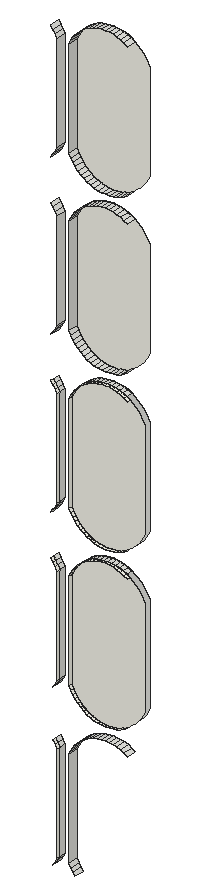
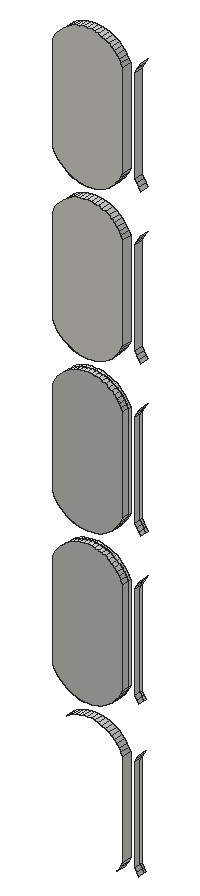
# SketchUp Ruby script. Lengths in inches.
U = 1.inch
M = Sketchup.active_model
def pt(a) = Geom::Point3d.new(a.map { |v| v * U })
def face(e, loops, mat)
  f = e.add_face(loops[0].map { |a| pt(a) })
  loops[1..].each { |l| e.add_face(l.map { |a| pt(a) }).erase! }
  f.material = f.back_material = mat if mat
  f
end
# faces: each face lists its corners as indices into pts; further lists are holes
def faces(e, pts, list, mat = nil) = list.each { |f| face(e, (f[0].is_a?(Array) ? f : [f]).map { |l| l.map { |i| pts[i] } }, mat) }
# xy, xz, yz: faces in a plane at the given z, y or x. An outline is a flat list of corners, or four numbers for a rectangle; further outlines are holes
def ring(l) = l.size == 4 ? [[l[0], l[1]], [l[2], l[1]], [l[2], l[3]], [l[0], l[3]]] : l.each_slice(2).to_a
def flat(e, list, mat, &to3) = list.each { |f| face(e, (f[0].is_a?(Array) ? f : [f]).map { |l| ring(l).map { |u, v| to3.(u, v) } }, mat) }
def xy(e, z, list, mat = nil) = flat(e, list, mat) { |x, y| [x, y, z] }
def xz(e, y, list, mat = nil) = flat(e, list, mat) { |x, z| [x, y, z] }
def yz(e, x, list, mat = nil) = flat(e, list, mat) { |y, z| [x, y, z] }
def lines(e, pts, list) = list.each { |a, b| e.add_line(pt(pts[a]), pt(pts[b])) }
# prism: a flat outline (further loops are holes) pulled along v
def prism(e, loops, v, mat = nil)
  f = face(e, loops, mat); d = Geom::Vector3d.new(v.map { |x| x * U })
  f.pushpull(f.normal.samedirection?(d) ? d.length : -d.length)
end
def box(e, o, s, mat = nil) = prism(e, [[o, [o[0] + s[0], o[1], o[2]], [o[0] + s[0], o[1] + s[1], o[2]], [o[0], o[1] + s[1], o[2]]]], [0, 0, s[2]], mat)
def at(x, y, z, deg = 0) = Geom::Transformation.translation(pt([x, y, z])) * Geom::Transformation.rotation(ORIGIN, Z_AXIS, deg.degrees)
def axes(o, x, y, z) = Geom::Transformation.new([*x, 0, *y, 0, *z, 0, *pt(o).to_a, 1])
def part(name) = M.definitions.add(name)
# library, detail: a bought-in or finely detailed component or shape, given as its bounding box
def library(name, o, s) = part(name).tap { |d| box(d.entities, o, s) }
def detail(e, o, s) = box(e.add_group.entities, o, s)
def put(e, d, t, mat = nil) = e.add_instance(d, t).tap { |i| i.material = mat if mat }
def group(e, t, mat = nil) = e.add_group.tap { |g| g.transformation = t; g.material = mat if mat }.entities
root = M.entities
M.materials.add("Tafisa-Gardenia-or-Gardenia-PM775-4K").color = [246, 245, 235]
xz(root,138.25,[[96.53,63,96.85,63.02,97.16,63.0625,97.47,63.14,97.76,63.25,98.05,63.38,98.32,63.55,98.57,63.74,98.81,63.95,99.02,64.19,99.21,64.44,99.37,64.71,99.5,65,99.5,73,99.37,73.29,99.21,73.56,99.02,73.81,98.81,74.05,98.57,74.26,98.32,74.45,98.05,74.62,97.76,74.75,97.47,74.86,97.16,74.9375,96.85,74.98,96.53,75,96.22,74.98,95.9,74.9375,95.6,74.86,95.3,74.75,95.01,74.62,94.74,74.45,94.49,74.26,94.25,74.05,94.04,73.81,93.86,73.56,93.7,73.29,93.5625,73,93.5625,65,93.7,64.71,93.86,64.44,94.04,64.19,94.25,63.95,94.49,63.74,94.74,63.55,95.01,63.38,95.3,63.25,95.6,63.14,95.9,63.0625,96.22,63.02],[96.53,76,96.85,76.02,97.16,76.0625,97.47,76.14,97.76,76.25,98.05,76.38,98.32,76.55,98.57,76.74,98.81,76.95,99.02,77.19,99.21,77.44,99.37,77.71,99.5,78,99.5,86,99.37,86.29,99.21,86.56,99.02,86.81,98.81,87.05,98.57,87.26,98.32,87.45,98.05,87.62,97.76,87.75,97.47,87.86,97.16,87.9375,96.85,87.98,96.53,88,96.22,87.98,95.9,87.9375,95.6,87.86,95.3,87.75,95.01,87.62,94.74,87.45,94.49,87.26,94.25,87.05,94.04,86.81,93.86,86.56,93.7,86.29,93.5625,86,93.5625,78,93.7,77.71,93.86,77.44,94.04,77.19,94.25,76.95,94.49,76.74,94.74,76.55,95.01,76.38,95.3,76.25,95.6,76.14,95.9,76.0625,96.22,76.02]],"Tafisa-Gardenia-or-Gardenia-PM775-4K")
xz(root,138.79,[[96.53,63,96.85,63.02,97.16,63.0625,97.47,63.14,97.76,63.25,98.05,63.38,98.32,63.55,98.57,63.74,98.81,63.95,99.02,64.19,99.21,64.44,99.37,64.71,99.5,65,99.5,73,99.37,73.29,99.21,73.56,99.02,73.81,98.81,74.05,98.57,74.26,98.32,74.45,98.05,74.62,97.76,74.75,97.47,74.86,97.16,74.9375,96.85,74.98,96.53,75,96.22,74.98,95.9,74.9375,95.6,74.86,95.3,74.75,95.01,74.62,94.74,74.45,94.49,74.26,94.25,74.05,94.04,73.81,93.86,73.56,93.7,73.29,93.5625,73,93.5625,65,93.7,64.71,93.86,64.44,94.04,64.19,94.25,63.95,94.49,63.74,94.74,63.55,95.01,63.38,95.3,63.25,95.6,63.14,95.9,63.0625,96.22,63.02],[96.53,76,96.85,76.02,97.16,76.0625,97.47,76.14,97.76,76.25,98.05,76.38,98.32,76.55,98.57,76.74,98.81,76.95,99.02,77.19,99.21,77.44,99.37,77.71,99.5,78,99.5,86,99.37,86.29,99.21,86.56,99.02,86.81,98.81,87.05,98.57,87.26,98.32,87.45,98.05,87.62,97.76,87.75,97.47,87.86,97.16,87.9375,96.85,87.98,96.53,88,96.22,87.98,95.9,87.9375,95.6,87.86,95.3,87.75,95.01,87.62,94.74,87.45,94.49,87.26,94.25,87.05,94.04,86.81,93.86,86.56,93.7,86.29,93.5625,86,93.5625,78,93.7,77.71,93.86,77.44,94.04,77.19,94.25,76.95,94.49,76.74,94.74,76.55,95.01,76.38,95.3,76.25,95.6,76.14,95.9,76.0625,96.22,76.02]])
xz(root,138.79,[[96.53,89,96.85,89.02,97.16,89.0625,97.47,89.14,97.76,89.25,98.05,89.38,98.32,89.55,98.57,89.74,98.81,89.95,99.02,90.19,99.21,90.44,99.37,90.71,99.5,91,99.5,99,99.37,99.29,99.21,99.56,99.02,99.81,98.81,100.05,98.57,100.26,98.32,100.45,98.05,100.62,97.76,100.75,97.47,100.86,97.16,100.9375,96.85,100.98,96.53,101,96.22,100.98,95.9,100.9375,95.6,100.86,95.3,100.75,95.01,100.62,94.74,100.45,94.49,100.26,94.25,100.05,94.04,99.81,93.86,99.56,93.7,99.29,93.5625,99,93.5625,91,93.7,90.71,93.86,90.44,94.04,90.19,94.25,89.95,94.49,89.74,94.74,89.55,95.01,89.38,95.3,89.25,95.6,89.14,95.9,89.0625,96.22,89.02],[96.53,102,96.85,102.02,97.16,102.0625,97.47,102.14,97.76,102.25,98.05,102.38,98.32,102.55,98.57,102.74,98.81,102.95,99.02,103.19,99.21,103.44,99.37,103.71,99.5,104,99.5,112,99.37,112.29,99.21,112.56,99.02,112.81,98.81,113.05,98.57,113.26,98.32,113.45,98.05,113.62,97.76,113.75,97.47,113.86,97.16,113.9375,96.85,113.98,96.53,114,96.22,113.98,95.9,113.9375,95.6,113.86,95.3,113.75,95.01,113.62,94.74,113.45,94.49,113.26,94.25,113.05,94.04,112.81,93.86,112.56,93.7,112.29,93.5625,112,93.5625,104,93.7,103.71,93.86,103.44,94.04,103.19,94.25,102.95,94.49,102.74,94.74,102.55,95.01,102.38,95.3,102.25,95.6,102.14,95.9,102.0625,96.22,102.02]],"Tafisa-Gardenia-or-Gardenia-PM775-4K")
yz(root,92.5625,[[138.25,52,138.79,60],[138.25,65,138.79,73],[138.25,78,138.79,86],[138,91,138.79,99],[138,104,138.79,112]])
yz(root,92.5625,[[138,52,138.25,60],[138,65,138.25,73],[138,78,138.25,86]],"Tafisa-Gardenia-or-Gardenia-PM775-4K")
yz(root,93.5625,[[138,52,138.79,60],[138.25,65,138.79,73],[138.25,78,138.79,86],[138,91,138.79,99],[138,104,138.79,112]])
yz(root,93.5625,[[138,65,138.25,73],[138,78,138.25,86]],"Tafisa-Gardenia-or-Gardenia-PM775-4K")
p = [[94.04,138.79,51.19],[93.86,138.79,51.44],[93.86,138,51.44],[94.04,138,51.19],[92.25,138,51.4375],[92.42,138,51.71],
  [92.42,138.25,51.71],[92.25,138.25,51.4375],[93.7,138.79,51.71],[93.7,138,51.71],[92.42,138.79,51.71],[92.25,138.79,51.4375],
  [92.5625,138,52],[92.5625,138.25,52],[93.5625,138.79,52],[93.5625,138,52],[92.5625,138.79,52],[92.5625,138,60],
  [92.42,138,60.29],[92.42,138.25,60.29],[92.5625,138.25,60],[93.5625,138.79,60],[93.7,138.79,60.29],[93.7,138,60.29],
  [93.5625,138,60],[92.42,138.79,60.29],[92.5625,138.79,60],[92.25,138,60.5625],[92.25,138.25,60.5625],[93.86,138.79,60.56],
  [93.86,138,60.56],[92.25,138.79,60.5625],[94.04,138.79,60.81],[94.04,138,60.81],[94.25,138.79,61.05],[94.25,138,61.05],
  [94.49,138.79,61.26],[94.49,138,61.26],[94.74,138.79,61.45],[94.74,138,61.45],[95.01,138.79,61.62],[95.01,138,61.62],
  [98.05,138.79,61.62],[98.32,138.79,61.45],[98.32,138,61.45],[98.05,138,61.62],[95.3,138.79,61.75],[95.3,138,61.75],
  [97.76,138.79,61.75],[97.76,138,61.75],[95.6,138.79,61.86],[95.6,138,61.86],[97.47,138.79,61.86],[97.47,138,61.86],
  [95.9,138.79,61.9375],[95.9,138,61.9375],[96.22,138.79,61.98],[96.22,138,61.98],[96.85,138.79,61.98],[97.16,138.79,61.9375],
  [97.16,138,61.9375],[96.85,138,61.98],[96.53,138.79,62],[96.53,138,62],[95.9,138,63.0625],[96.22,138,63.02],
  [96.22,138.25,63.02],[95.9,138.25,63.0625],[96.53,138,63],[96.53,138.25,63],[96.85,138,63.02],[96.85,138.25,63.02],
  [97.16,138,63.0625],[97.16,138.25,63.0625],[96.22,138.79,63.02],[95.9,138.79,63.0625],[96.53,138.79,63],[96.85,138.79,63.02],
  [97.16,138.79,63.0625],[95.3,138,63.25],[95.6,138,63.14],[95.6,138.25,63.14],[95.3,138.25,63.25],[97.47,138,63.14],
  [97.47,138.25,63.14],[97.76,138,63.25],[97.76,138.25,63.25],[95.6,138.79,63.14],[95.3,138.79,63.25],[97.47,138.79,63.14],
  [97.76,138.79,63.25],[95.01,138,63.38],[95.01,138.25,63.38],[98.05,138,63.38],[98.05,138.25,63.38],[95.01,138.79,63.38],
  [98.05,138.79,63.38],[94.74,138,63.55],[94.74,138.25,63.55],[98.32,138,63.55],[98.32,138.25,63.55],[94.74,138.79,63.55],
  [98.32,138.79,63.55],[94.49,138,63.74],[94.49,138.25,63.74],[94.49,138.79,63.74],[94.25,138,63.95],[94.25,138.25,63.95],
  [94.25,138.79,63.95],[94.04,138,64.19],[94.04,138.25,64.19],[94.04,138.79,64.19],[93.86,138,64.44],[93.86,138.25,64.44],
  [93.86,138.79,64.44],[92.25,138,64.4375],[92.42,138,64.71],[92.42,138.25,64.71],[92.25,138.25,64.4375],[93.7,138,64.71],
  [93.7,138.25,64.71],[92.42,138.79,64.71],[92.25,138.79,64.4375],[93.7,138.79,64.71],[92.5625,138,65],[92.5625,138.25,65],
  [93.5625,138,65],[93.5625,138.25,65],[92.5625,138.79,65],[93.5625,138.79,65],[92.5625,138,73],[92.42,138,73.29],
  [92.42,138.25,73.29],[92.5625,138.25,73],[93.7,138,73.29],[93.5625,138,73],[93.5625,138.25,73],[93.7,138.25,73.29],
  [92.42,138.79,73.29],[92.5625,138.79,73],[93.5625,138.79,73],[93.7,138.79,73.29],[92.25,138,73.5625],[92.25,138.25,73.5625],
  [93.86,138,73.56],[93.86,138.25,73.56],[92.25,138.79,73.5625],[93.86,138.79,73.56],[92.0625,138,73.82],[92.0625,138.25,73.82],
  [94.04,138,73.81],[94.04,138.25,73.81],[92.0625,138.79,73.82],[94.04,138.79,73.81],[94.25,138,74.05],[94.25,138.25,74.05],
  [94.25,138.79,74.05],[94.49,138,74.26],[94.49,138.25,74.26],[94.49,138.79,74.26],[94.74,138,74.45],[94.74,138.25,74.45],
  [94.74,138.79,74.45],[95.01,138,74.62],[95.01,138.25,74.62],[98.32,138,74.45],[98.05,138,74.62],[98.05,138.25,74.62],
  [98.32,138.25,74.45],[95.01,138.79,74.62],[95.3,138,74.75],[95.3,138.25,74.75],[97.76,138,74.75],[97.76,138.25,74.75],
  [95.3,138.79,74.75],[97.76,138.79,74.75],[98.05,138.79,74.62],[95.6,138,74.86],[95.6,138.25,74.86],[97.47,138,74.86],
  [97.47,138.25,74.86],[95.6,138.79,74.86],[97.47,138.79,74.86],[95.9,138,74.9375],[95.9,138.25,74.9375],[96.22,138,74.98],
  [96.22,138.25,74.98],[97.16,138,74.9375],[96.85,138,74.98],[96.85,138.25,74.98],[97.16,138.25,74.9375],[95.9,138.79,74.9375],
  [96.22,138.79,74.98],[96.85,138.79,74.98],[97.16,138.79,74.9375],[96.53,138,75],[96.53,138.25,75],[96.53,138.79,75],
  [95.9,138,76.0625],[96.22,138,76.02],[96.22,138.25,76.02],[95.9,138.25,76.0625],[96.53,138,76],[96.53,138.25,76],
  [96.85,138,76.02],[96.85,138.25,76.02],[97.16,138,76.0625],[97.16,138.25,76.0625],[96.22,138.79,76.02],[95.9,138.79,76.0625],
  [96.53,138.79,76],[96.85,138.79,76.02],[97.16,138.79,76.0625],[95.3,138,76.25],[95.6,138,76.14],[95.6,138.25,76.14],
  [95.3,138.25,76.25],[97.47,138,76.14],[97.47,138.25,76.14],[97.76,138,76.25],[97.76,138.25,76.25],[95.6,138.79,76.14],
  [95.3,138.79,76.25],[97.47,138.79,76.14],[97.76,138.79,76.25],[95.01,138,76.38],[95.01,138.25,76.38],[98.05,138,76.38],
  [98.05,138.25,76.38],[95.01,138.79,76.38],[98.05,138.79,76.38],[94.74,138,76.55],[94.74,138.25,76.55],[98.32,138,76.55],
  [98.32,138.25,76.55],[94.74,138.79,76.55],[94.49,138,76.74],[94.49,138.25,76.74],[94.49,138.79,76.74],[94.25,138,76.95],
  [94.25,138.25,76.95],[94.25,138.79,76.95],[94.04,138,77.19],[94.04,138.25,77.19],[94.04,138.79,77.19],[92.0625,138,77.18],
  [92.25,138,77.4375],[92.25,138.25,77.4375],[92.0625,138.25,77.18],[93.86,138,77.44],[93.86,138.25,77.44],[92.25,138.79,77.4375],
  [92.0625,138.79,77.18],[93.86,138.79,77.44],[92.42,138,77.71],[92.42,138.25,77.71],[93.7,138,77.71],[93.7,138.25,77.71],
  [92.42,138.79,77.71],[93.7,138.79,77.71],[92.5625,138,78],[92.5625,138.25,78],[93.5625,138,78],[93.5625,138.25,78],
  [92.5625,138.79,78],[93.5625,138.79,78],[92.5625,138,86],[92.42,138,86.29],[92.42,138.25,86.29],[92.5625,138.25,86],
  [93.7,138,86.29],[93.5625,138,86],[93.5625,138.25,86],[93.7,138.25,86.29],[92.42,138.79,86.29],[92.5625,138.79,86],
  [93.5625,138.79,86],[93.7,138.79,86.29],[92.25,138,86.5625],[92.25,138.25,86.5625],[93.86,138,86.56],[93.86,138.25,86.56],
  [92.25,138.79,86.5625],[93.86,138.79,86.56],[92.0625,138,86.82],[92.0625,138.25,86.82],[94.04,138,86.81],[94.04,138.25,86.81],
  [92.0625,138.79,86.82],[94.04,138.79,86.81],[94.25,138,87.05],[94.25,138.25,87.05],[94.25,138.79,87.05],[94.49,138,87.26],
  [94.49,138.25,87.26],[94.49,138.79,87.26],[94.74,138,87.45],[94.74,138.25,87.45],[94.74,138.79,87.45],[95.01,138,87.62],
  [95.01,138.25,87.62],[98.32,138,87.45],[98.05,138,87.62],[98.05,138.25,87.62],[98.32,138.25,87.45],[95.01,138.79,87.62],
  [95.3,138,87.75],[95.3,138.25,87.75],[97.76,138,87.75],[97.76,138.25,87.75],[95.3,138.79,87.75],[97.76,138.79,87.75],
  [98.05,138.79,87.62],[95.6,138,87.86],[95.6,138.25,87.86],[97.47,138,87.86],[97.47,138.25,87.86],[95.6,138.79,87.86],
  [97.47,138.79,87.86],[95.9,138,87.9375],[95.9,138.25,87.9375],[96.22,138,87.98],[96.22,138.25,87.98],[97.16,138,87.9375],
  [96.85,138,87.98],[96.85,138.25,87.98],[97.16,138.25,87.9375],[95.9,138.79,87.9375],[96.22,138.79,87.98],[96.85,138.79,87.98],
  [97.16,138.79,87.9375],[96.53,138,88],[96.53,138.25,88],[96.53,138.79,88],[96.22,138.79,89.02],[95.9,138.79,89.0625],
  [95.9,138,89.0625],[96.22,138,89.02],[96.53,138.79,89],[96.53,138,89],[96.85,138.79,89.02],[96.85,138,89.02],
  [97.16,138.79,89.0625],[97.16,138,89.0625],[95.6,138.79,89.14],[95.3,138.79,89.25],[95.3,138,89.25],[95.6,138,89.14],
  [97.47,138.79,89.14],[97.47,138,89.14],[97.76,138.79,89.25],[97.76,138,89.25],[95.01,138.79,89.38],[95.01,138,89.38],
  [98.05,138.79,89.38],[98.05,138,89.38],[94.74,138.79,89.55],[94.74,138,89.55],[98.32,138.79,89.55],[98.32,138,89.55],
  [94.49,138.79,89.74],[94.49,138,89.74],[94.25,138.79,89.95],[94.25,138,89.95],[94.04,138.79,90.19],[94.04,138,90.19],
  [92.25,138.79,90.4375],[92.0625,138.79,90.18],[92.0625,138,90.18],[92.25,138,90.4375],[93.86,138.79,90.44],[93.86,138,90.44],
  [92.42,138.79,90.71],[92.42,138,90.71],[93.7,138.79,90.71],[93.7,138,90.71],[92.5625,138.79,91],[92.5625,138,91],
  [93.5625,138.79,91],[93.5625,138,91],[92.42,138.79,99.29],[92.5625,138.79,99],[92.5625,138,99],[92.42,138,99.29],
  [93.5625,138.79,99],[93.7,138.79,99.29],[93.7,138,99.29],[93.5625,138,99],[92.25,138.79,99.5625],[92.25,138,99.5625],
  [93.86,138.79,99.56],[93.86,138,99.56],[92.0625,138.79,99.82],[92.0625,138,99.82],[94.04,138.79,99.81],[94.04,138,99.81],
  [94.25,138.79,100.05],[94.25,138,100.05],[94.49,138.79,100.26],[94.49,138,100.26],[94.74,138.79,100.45],[94.74,138,100.45],
  [95.01,138.79,100.62],[95.01,138,100.62],[98.05,138.79,100.62],[98.32,138.79,100.45],[98.32,138,100.45],[98.05,138,100.62],
  [95.3,138.79,100.75],[95.3,138,100.75],[97.76,138.79,100.75],[97.76,138,100.75],[95.6,138.79,100.86],[95.6,138,100.86],
  [97.47,138.79,100.86],[97.47,138,100.86],[95.9,138.79,100.9375],[95.9,138,100.9375],[96.22,138.79,100.98],[96.22,138,100.98],
  [96.85,138.79,100.98],[97.16,138.79,100.9375],[97.16,138,100.9375],[96.85,138,100.98],[96.53,138.79,101],[96.53,138,101],
  [96.22,138.79,102.02],[95.9,138.79,102.0625],[95.9,138,102.0625],[96.22,138,102.02],[96.53,138.79,102],[96.53,138,102],
  [96.85,138.79,102.02],[96.85,138,102.02],[97.16,138.79,102.0625],[97.16,138,102.0625],[95.6,138.79,102.14],[95.3,138.79,102.25],
  [95.3,138,102.25],[95.6,138,102.14],[97.47,138.79,102.14],[97.47,138,102.14],[97.76,138.79,102.25],[97.76,138,102.25],
  [95.01,138.79,102.38],[95.01,138,102.38],[98.05,138.79,102.38],[98.05,138,102.38],[94.74,138.79,102.55],[94.74,138,102.55],
  [98.32,138.79,102.55],[98.32,138,102.55],[94.49,138.79,102.74],[94.49,138,102.74],[94.25,138.79,102.95],[94.25,138,102.95],
  [94.04,138.79,103.19],[94.04,138,103.19],[92.25,138.79,103.4375],[92.0625,138.79,103.18],[92.0625,138,103.18],[92.25,138,103.4375],
  [93.86,138.79,103.44],[93.86,138,103.44],[92.42,138.79,103.71],[92.42,138,103.71],[93.7,138.79,103.71],[93.7,138,103.71],
  [92.5625,138.79,104],[92.5625,138,104],[93.5625,138.79,104],[93.5625,138,104],[92.42,138.79,112.29],[92.5625,138.79,112],
  [92.5625,138,112],[92.42,138,112.29],[93.5625,138.79,112],[93.7,138.79,112.29],[93.7,138,112.29],[93.5625,138,112],
  [92.25,138.79,112.5625],[92.25,138,112.5625],[93.86,138.79,112.56],[93.86,138,112.56],[92.0625,138.79,112.82],[92.0625,138,112.82],
  [94.04,138.79,112.81],[94.04,138,112.81],[94.25,138.79,113.05],[94.25,138,113.05],[94.49,138.79,113.26],[94.49,138,113.26],
  [94.74,138.79,113.45],[94.74,138,113.45],[95.01,138.79,113.62],[95.01,138,113.62],[98.05,138.79,113.62],[98.32,138.79,113.45],
  [98.32,138,113.45],[98.05,138,113.62],[95.3,138.79,113.75],[95.3,138,113.75],[97.76,138.79,113.75],[97.76,138,113.75],
  [95.6,138.79,113.86],[95.6,138,113.86],[97.47,138.79,113.86],[97.47,138,113.86],[95.9,138.79,113.9375],[95.9,138,113.9375],
  [96.22,138.79,113.98],[96.22,138,113.98],[96.85,138.79,113.98],[97.16,138.79,113.9375],[97.16,138,113.9375],[96.85,138,113.98],
  [96.53,138.79,114],[96.53,138,114]]
faces(root,p,[[0,1,2,3],[1,8,9,2],[10,11,7,6],[8,14,15,9],[16,10,6,13],[21,22,23,24],[25,26,20,19],[22,29,30,23],
  [31,25,19,28],[29,32,33,30],[32,34,35,33],[34,36,37,35],[36,38,39,37],[38,40,41,39],[42,43,44,45],[40,46,47,41],
  [48,42,45,49],[46,50,51,47],[52,48,49,53],[50,54,55,51],[54,56,57,55],[58,59,60,61],[59,52,53,60],[56,62,63,57],
  [62,58,61,63],[74,75,67,66],[76,74,66,69],[77,76,69,71],[78,77,71,73],[87,88,82,81],[75,87,81,67],[89,78,73,84],
  [90,89,84,86],[88,95,92,82],[96,90,86,94],[95,101,98,92],[102,96,94,100],[101,105,104,98],[105,108,107,104],[108,111,110,107],
  [111,114,113,110],[121,122,118,117],[114,123,120,113],[128,121,117,125],[123,129,127,120],[138,139,133,132],[140,141,137,136],[146,138,132,143],
  [141,147,145,137],[152,146,143,149],[147,153,151,145],[153,156,155,151],[156,159,158,155],[159,162,161,158],[162,169,164,161],[169,174,171,164],
  [175,176,167,173],[174,181,178,171],[182,175,173,180],[181,191,184,178],[191,192,186,184],[193,194,190,189],[194,182,180,190],[192,197,196,186],
  [197,193,189,196],[208,209,201,200],[210,208,200,203],[211,210,203,205],[212,211,205,207],[221,222,216,215],[209,221,215,201],[223,212,207,218],
  [224,223,218,220],[222,229,226,216],[230,224,220,228],[229,235,232,226],[235,238,237,232],[238,241,240,237],[241,244,243,240],[251,252,248,247],
  [244,253,250,243],[258,251,247,255],[253,259,257,250],[264,258,255,261],[259,265,263,257],[274,275,269,268],[276,277,273,272],[282,274,268,279],
  [277,283,281,273],[288,282,279,285],[283,289,287,281],[289,292,291,287],[292,295,294,291],[295,298,297,294],[298,305,300,297],[305,310,307,300],
  [311,312,303,309],[310,317,314,307],[318,311,309,316],[317,327,320,314],[327,328,322,320],[329,330,326,325],[330,318,316,326],[328,333,332,322],
  [333,329,325,332],[334,335,336,337],[338,334,337,339],[340,338,339,341],[342,340,341,343],[344,345,346,347],[335,344,347,336],[348,342,343,349],
  [350,348,349,351],[345,352,353,346],[354,350,351,355],[352,356,357,353],[358,354,355,359],[356,360,361,357],[360,362,363,361],[362,364,365,363],
  [366,367,368,369],[364,370,371,365],[372,366,369,373],[370,374,375,371],[376,372,373,377],[374,378,379,375],[380,381,382,383],[384,385,386,387],
  [388,380,383,389],[385,390,391,386],[392,388,389,393],[390,394,395,391],[394,396,397,395],[396,398,399,397],[398,400,401,399],[400,402,403,401],
  [404,405,406,407],[402,408,409,403],[410,404,407,411],[408,412,413,409],[414,410,411,415],[412,416,417,413],[416,418,419,417],[420,421,422,423],
  [421,414,415,422],[418,424,425,419],[424,420,423,425],[426,427,428,429],[430,426,429,431],[432,430,431,433],[434,432,433,435],[436,437,438,439],
  [427,436,439,428],[440,434,435,441],[442,440,441,443],[437,444,445,438],[446,442,443,447],[444,448,449,445],[450,446,447,451],[448,452,453,449],
  [452,454,455,453],[454,456,457,455],[458,459,460,461],[456,462,463,457],[464,458,461,465],[462,466,467,463],[468,464,465,469],[466,470,471,467],
  [472,473,474,475],[476,477,478,479],[480,472,475,481],[477,482,483,478],[484,480,481,485],[482,486,487,483],[486,488,489,487],[488,490,491,489],
  [490,492,493,491],[492,494,495,493],[496,497,498,499],[494,500,501,495],[502,496,499,503],[500,504,505,501],[506,502,503,507],[504,508,509,505],
  [508,510,511,509],[512,513,514,515],[513,506,507,514],[510,516,517,511],[516,512,515,517]])
faces(root,p,[[4,5,6,7],[5,12,13,6],[17,18,19,20],[18,27,28,19],[64,65,66,67],[65,68,69,66],[68,70,71,69],[70,72,73,71],
  [79,80,81,82],[80,64,67,81],[72,83,84,73],[83,85,86,84],[91,79,82,92],[85,93,94,86],[97,91,92,98],[93,99,100,94],
  [103,97,98,104],[106,103,104,107],[109,106,107,110],[112,109,110,113],[115,116,117,118],[119,112,113,120],[116,124,125,117],[126,119,120,127],
  [130,131,132,133],[134,135,136,137],[131,142,143,132],[144,134,137,145],[142,148,149,143],[150,144,145,151],[154,150,151,155],[157,154,155,158],
  [160,157,158,161],[163,160,161,164],[165,166,167,168],[170,163,164,171],[166,172,173,167],[177,170,171,178],[172,179,180,173],[183,177,178,184],
  [185,183,184,186],[187,188,189,190],[179,187,190,180],[195,185,186,196],[188,195,196,189],[198,199,200,201],[199,202,203,200],[202,204,205,203],
  [204,206,207,205],[213,214,215,216],[214,198,201,215],[206,217,218,207],[217,219,220,218],[225,213,216,226],[219,227,228,220],[231,225,226,232],
  [227,233,234,228],[236,231,232,237],[239,236,237,240],[242,239,240,243],[245,246,247,248],[249,242,243,250],[246,254,255,247],[256,249,250,257],
  [254,260,261,255],[262,256,257,263],[266,267,268,269],[270,271,272,273],[267,278,279,268],[280,270,273,281],[278,284,285,279],[286,280,281,287],
  [290,286,287,291],[293,290,291,294],[296,293,294,297],[299,296,297,300],[301,302,303,304],[306,299,300,307],[302,308,309,303],[313,306,307,314],
  [308,315,316,309],[319,313,314,320],[321,319,320,322],[323,324,325,326],[315,323,326,316],[331,321,322,332],[324,331,332,325]],"Tafisa-Gardenia-or-Gardenia-PM775-4K")
